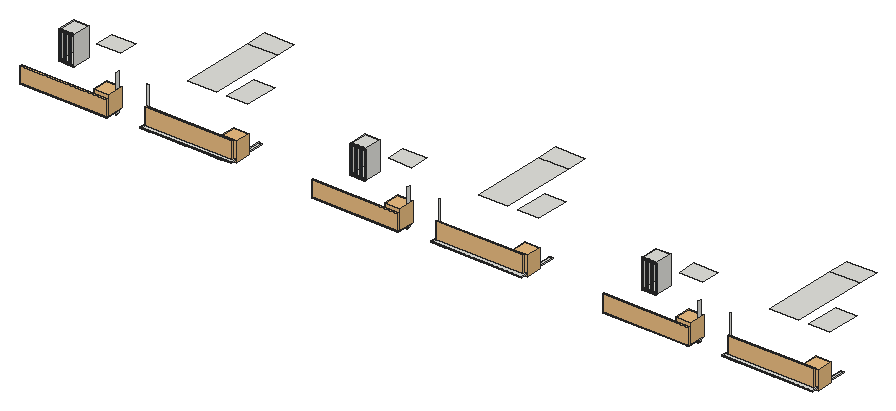
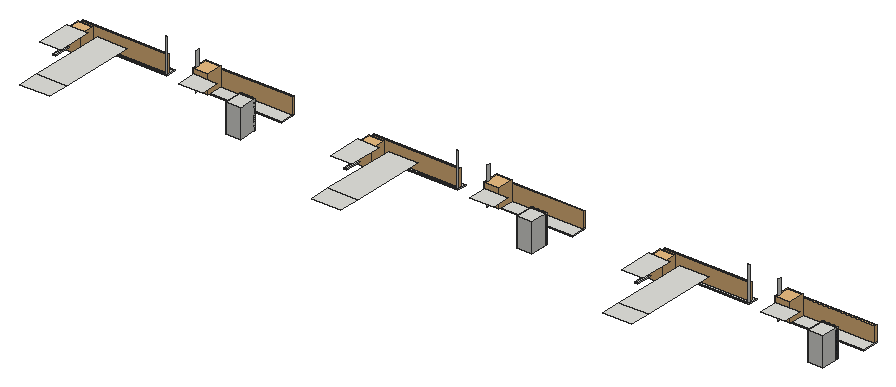
# SketchUp Ruby script. Lengths in inches.
U = 1.inch
M = Sketchup.active_model
def pt(a) = Geom::Point3d.new(a.map { |v| v * U })
def face(e, loops, mat)
  f = e.add_face(loops[0].map { |a| pt(a) })
  loops[1..].each { |l| e.add_face(l.map { |a| pt(a) }).erase! }
  f.material = f.back_material = mat if mat
  f
end
# faces: each face lists its corners as indices into pts; further lists are holes
def faces(e, pts, list, mat = nil) = list.each { |f| face(e, (f[0].is_a?(Array) ? f : [f]).map { |l| l.map { |i| pts[i] } }, mat) }
# xy, xz, yz: faces in a plane at the given z, y or x. An outline is a flat list of corners, or four numbers for a rectangle; further outlines are holes
def ring(l) = l.size == 4 ? [[l[0], l[1]], [l[2], l[1]], [l[2], l[3]], [l[0], l[3]]] : l.each_slice(2).to_a
def flat(e, list, mat, &to3) = list.each { |f| face(e, (f[0].is_a?(Array) ? f : [f]).map { |l| ring(l).map { |u, v| to3.(u, v) } }, mat) }
def xy(e, z, list, mat = nil) = flat(e, list, mat) { |x, y| [x, y, z] }
def xz(e, y, list, mat = nil) = flat(e, list, mat) { |x, z| [x, y, z] }
def yz(e, x, list, mat = nil) = flat(e, list, mat) { |y, z| [x, y, z] }
def lines(e, pts, list) = list.each { |a, b| e.add_line(pt(pts[a]), pt(pts[b])) }
# prism: a flat outline (further loops are holes) pulled along v
def prism(e, loops, v, mat = nil)
  f = face(e, loops, mat); d = Geom::Vector3d.new(v.map { |x| x * U })
  f.pushpull(f.normal.samedirection?(d) ? d.length : -d.length)
end
def box(e, o, s, mat = nil) = prism(e, [[o, [o[0] + s[0], o[1], o[2]], [o[0] + s[0], o[1] + s[1], o[2]], [o[0], o[1] + s[1], o[2]]]], [0, 0, s[2]], mat)
def at(x, y, z, deg = 0) = Geom::Transformation.translation(pt([x, y, z])) * Geom::Transformation.rotation(ORIGIN, Z_AXIS, deg.degrees)
def axes(o, x, y, z) = Geom::Transformation.new([*x, 0, *y, 0, *z, 0, *pt(o).to_a, 1])
def part(name) = M.definitions.add(name)
# library, detail: a bought-in or finely detailed component or shape, given as its bounding box
def library(name, o, s) = part(name).tap { |d| box(d.entities, o, s) }
def detail(e, o, s) = box(e.add_group.entities, o, s)
def put(e, d, t, mat = nil) = e.add_instance(d, t).tap { |i| i.material = mat if mat }
def group(e, t, mat = nil) = e.add_group.tap { |g| g.transformation = t; g.material = mat if mat }.entities
root = M.entities
M.materials.add("Wine2").color = [0, 0, 0]
M.materials["Wine2"].alpha = 0
M.materials.add("[0130_Gainsboro]").color = [39, 45, 50]
M.materials.add("[Wood Veneer 01]").color = [51, 28, 15]
c1 = library("plant (1)",[-35.72,-28.42,0],[66.31,67.39,84.38])
c2 = library("Glass Railing",[0,0,0],[139.5,4.76,42])
c3 = part("Group\#55")
xy(c3.entities,0,[[0,-0.98,43.07,0],[0,0,43.07,1.4]],"[0130_Gainsboro]")
xy(c3.entities,0.3,[[0.3,-1.43,42.77,-0.98]],"[0130_Gainsboro]")
xy(c3.entities,2.95,[[2.95,-1.43,40.12,-0.63],[2.95,-0.63,40.12,0],[2.95,0,40.12,0.64],[2.95,0.64,40.12,1.4]],"[0130_Gainsboro]")
xy(c3.entities,3.54,[[3.54,-0.63,39.53,0],[3.54,0,39.53,0.64]],"[0130_Gainsboro]")
xy(c3.entities,111.8125,[[3.54,-0.63,39.53,0],[3.54,0,39.53,0.64]],"[0130_Gainsboro]")
xy(c3.entities,112.4,[[2.95,-1.43,40.12,-0.63],[2.95,-0.63,40.12,0],[2.95,0,40.12,0.64],[2.95,0.64,40.12,1.4]],"[0130_Gainsboro]")
xy(c3.entities,115.05,[[0.3,-1.43,42.77,-0.98]],"[0130_Gainsboro]")
xy(c3.entities,115.35,[[0,-0.98,43.07,0],[0,0,43.07,1.4]],"[0130_Gainsboro]")
xz(c3.entities,-1.43,[[[0.3,0.3,42.77,115.05],[2.95,2.95,40.12,112.4]]],"[Wood Veneer 01]")
xz(c3.entities,-0.98,[[[0,0,43.07,115.35],[0.3,0.3,42.77,115.05]]],"[0130_Gainsboro]")
xz(c3.entities,-0.63,[[[2.95,2.95,40.12,112.4],[3.54,3.54,39.53,111.8125]]],"[0130_Gainsboro]")
xz(c3.entities,0,[[3.54,3.54,39.53,111.8125]],"Wine2")
xz(c3.entities,0,[[[0,0,43.07,115.35],[2.95,2.95,40.12,112.4]],[[2.95,2.95,40.12,112.4],[3.54,3.54,39.53,111.8125]]],"[0130_Gainsboro]")
xz(c3.entities,0.64,[[[2.95,2.95,40.12,112.4],[3.54,3.54,39.53,111.8125]]],"[0130_Gainsboro]")
xz(c3.entities,1.4,[[[0,0,43.07,115.35],[2.95,2.95,40.12,112.4]]],"[0130_Gainsboro]")
yz(c3.entities,0,[[-0.98,0,0,115.35],[0,0,1.4,115.35]],"[0130_Gainsboro]")
yz(c3.entities,0.3,[[-1.43,0.3,-0.98,115.05]],"[0130_Gainsboro]")
yz(c3.entities,2.95,[[-1.43,2.95,-0.63,112.4],[-0.63,2.95,0,112.4],[0,2.95,0.64,112.4],[0.64,2.95,1.4,112.4]],"[0130_Gainsboro]")
yz(c3.entities,3.54,[[-0.63,3.54,0,111.8125],[0,3.54,0.64,111.8125]],"[0130_Gainsboro]")
yz(c3.entities,39.53,[[-0.63,3.54,0,111.8125],[0,3.54,0.64,111.8125]],"[0130_Gainsboro]")
yz(c3.entities,40.12,[[-1.43,2.95,-0.63,112.4],[-0.63,2.95,0,112.4],[0,2.95,0.64,112.4],[0.64,2.95,1.4,112.4]],"[0130_Gainsboro]")
yz(c3.entities,42.77,[[-1.43,0.3,-0.98,115.05]],"[0130_Gainsboro]")
yz(c3.entities,43.07,[[-0.98,0,0,115.35],[0,0,1.4,115.35]],"[0130_Gainsboro]")
c4 = part("Component\#21")
put(c4.entities,c3,axes([90.57,1.43,0],[1.05148,0,0],[0,1,0],[0,0,1]))
put(c4.entities,c3,axes([0,1.43,0],[1.05148,0,0],[0,1,0],[0,0,1]))
put(c4.entities,c3,axes([45.29,1.43,0],[1.05148,0,0],[0,1,0],[0,0,1]),"[Wood Veneer 01]")
xy(root,409.375,[[315.43,286.21,315.68,293.45],[1049,286.21,1049.24,293.45],[1782.56,286.21,1782.8,293.45]])
xy(root,416.75,[[100.18,253.3,100.18,253.61,315.68,253.61,315.68,255.92,318.3,255.92,318.3,253.3],[833.74,253.3,833.74,253.61,1049.24,253.61,1049.24,255.92,1051.86,255.92,1051.86,253.3],[1567.3,253.3,1567.3,253.61,1782.8,253.61,1782.8,255.92,1785.43,255.92,1785.43,253.3],[100.18,253.61,315.68,293.45],[833.74,253.61,1049.24,293.45],
  [1567.3,253.61,1782.8,293.45],[315.68,255.92,318.3,293.45],[1049.24,255.92,1051.86,293.45],[1782.8,255.92,1785.43,293.45],[393.95,263.8,393.95,286.21,614.76,286.21,614.76,361.27,622,361.27,622,266.43,398.72,266.43,398.72,263.8],
  [398.72,263.8,404.72,266.43],[404.72,263.8,410.72,266.43],[410.72,263.8,416.72,266.43],[416.72,263.8,422.72,266.43],[422.72,263.8,428.72,266.43],
  [428.72,263.8,434.72,266.43],[434.72,263.8,440.72,266.43],[440.72,263.8,446.72,266.43],[446.72,263.8,452.72,266.43],[452.72,263.8,458.72,266.43],
  [458.72,263.8,464.72,266.43],[464.72,263.8,470.72,266.43],[470.72,263.8,476.72,266.43],[476.72,263.8,482.72,266.43],[482.72,263.8,488.72,266.43],
  [488.72,263.8,494.72,266.43],[494.72,263.8,500.72,266.43],[500.72,263.8,506.72,266.43],[506.72,263.8,512.72,266.43],[512.72,263.8,518.72,266.43],
  [518.72,263.8,524.72,266.43],[524.72,263.8,530.72,266.43],[530.72,263.8,536.72,266.43],[536.72,263.8,542.72,266.43],[542.72,263.8,548.72,266.43],
  [548.72,263.8,554.72,266.43],[554.72,263.8,560.72,266.43],[560.72,263.8,566.72,266.43],[566.72,263.8,572.72,266.43],[572.72,263.8,578.72,266.43],
  [578.72,263.8,584.72,266.43],[584.72,263.8,590.72,266.43],[590.72,263.8,596.72,266.43],[596.72,263.8,602.72,266.43],[602.72,263.8,608.72,266.43],
  [608.72,263.8,622,266.43],[1127.51,263.8,1127.51,286.21,1348.32,286.21,1348.32,361.27,1355.5625,361.27,1355.5625,266.43,1132.28,266.43,1132.28,263.8],[1132.28,263.8,1138.28,266.43],[1138.28,263.8,1144.28,266.43],[1144.28,263.8,1150.28,266.43],
  [1150.28,263.8,1156.28,266.43],[1156.28,263.8,1162.28,266.43],[1162.28,263.8,1168.28,266.43],[1168.28,263.8,1174.28,266.43],[1174.28,263.8,1180.28,266.43],
  [1180.28,263.8,1186.28,266.43],[1186.28,263.8,1192.28,266.43],[1192.28,263.8,1198.28,266.43],[1198.28,263.8,1204.28,266.43],[1204.28,263.8,1210.28,266.43],
  [1210.28,263.8,1216.28,266.43],[1216.28,263.8,1222.28,266.43],[1222.28,263.8,1228.28,266.43],[1228.28,263.8,1234.28,266.43],[1234.28,263.8,1240.28,266.43],
  [1240.28,263.8,1246.28,266.43],[1246.28,263.8,1252.28,266.43],[1252.28,263.8,1258.28,266.43],[1258.28,263.8,1264.28,266.43],[1264.28,263.8,1270.28,266.43],
  [1270.28,263.8,1276.28,266.43],[1276.28,263.8,1282.28,266.43],[1282.28,263.8,1288.28,266.43],[1288.28,263.8,1294.28,266.43],[1294.28,263.8,1300.28,266.43],
  [1300.28,263.8,1306.28,266.43],[1306.28,263.8,1312.28,266.43],[1312.28,263.8,1318.28,266.43],[1318.28,263.8,1324.28,266.43],[1324.28,263.8,1330.28,266.43],
  [1330.28,263.8,1336.28,266.43],[1336.28,263.8,1342.28,266.43],[1342.28,263.8,1355.5625,266.43],[1861.07,263.8,1861.07,286.21,2081.89,286.21,2081.89,361.27,2089.125,361.27,2089.125,266.43,1865.84,266.43,1865.84,263.8],[1865.84,263.8,1871.84,266.43],
  [1871.84,263.8,1877.84,266.43],[1877.84,263.8,1883.84,266.43],[1883.84,263.8,1889.84,266.43],[1889.84,263.8,1895.84,266.43],[1895.84,263.8,1901.84,266.43],
  [1901.84,263.8,1907.84,266.43],[1907.84,263.8,1913.84,266.43],[1913.84,263.8,1919.84,266.43],[1919.84,263.8,1925.84,266.43],[1925.84,263.8,1931.84,266.43],
  [1931.84,263.8,1937.84,266.43],[1937.84,263.8,1943.84,266.43],[1943.84,263.8,1949.84,266.43],[1949.84,263.8,1955.84,266.43],[1955.84,263.8,1961.84,266.43],
  [1961.84,263.8,1967.84,266.43],[1967.84,263.8,1973.84,266.43],[1973.84,263.8,1979.84,266.43],[1979.84,263.8,1985.84,266.43],[1985.84,263.8,1991.84,266.43],
  [1991.84,263.8,1997.84,266.43],[1997.84,263.8,2003.84,266.43],[2003.84,263.8,2009.84,266.43],[2009.84,263.8,2015.84,266.43],[2015.84,263.8,2021.84,266.43],
  [2021.84,263.8,2027.84,266.43],[2027.84,263.8,2033.84,266.43],[2033.84,263.8,2039.84,266.43],[2039.84,263.8,2045.84,266.43],[2045.84,263.8,2051.84,266.43],
  [2051.84,263.8,2057.84,266.43],[2057.84,263.8,2063.84,266.43],[2063.84,263.8,2069.84,266.43],[2069.84,263.8,2075.84,266.43],[2075.84,263.8,2089.125,266.43]])
xy(root,418.9375,[[100.18,253.3,318.3,293.45],[833.74,253.3,1051.86,293.45],[1567.3,253.3,1785.43,293.45],[393.95,263.8,622,263.8,622,361.27,614.76,361.27,614.76,286.21,393.95,286.21],[1127.51,263.8,1355.5625,263.8,1355.5625,361.27,1348.32,361.27,1348.32,286.21,1127.51,286.21],
  [1861.07,263.8,2089.125,263.8,2089.125,361.27,2081.89,361.27,2081.89,286.21,1861.07,286.21]])
xy(root,425.31,[[111.92,361.27,149.24,408.14],[845.49,361.27,882.8,408.14],[1579.05,361.27,1616.36,408.14]])
xy(root,495.625,[[435.49,361.27,509.74,551.2],[1169.05,361.27,1243.3,551.2],[1902.61,361.27,1976.86,551.2],[435.49,551.2,509.74,604.39],[1169.05,551.2,1243.3,604.39],
  [1902.61,551.2,1976.86,604.39]])
xy(root,495.6875,[[534.92,361.27,587.67,445.08],[1268.48,361.27,1321.23,445.08],[2002.05,361.27,2054.8,445.08]])
xy(root,497.42,[[207.81,361.27,266.47,408.14],[941.37,361.27,1000.03,408.14],[1674.93,361.27,1733.6,408.14]])
xy(root,497.43,[[111.92,361.27,149.24,408.14],[845.49,361.27,882.8,408.14],[1579.05,361.27,1616.36,408.14]])
xz(root,253.3,[[100.18,416.75,318.3,418.9375],[833.74,416.75,1051.86,418.9375],[1567.3,416.75,1785.43,418.9375]],"[Wood Veneer 01]")
xz(root,263.8,[[393.95,416.75,622,418.9375],[1127.51,416.75,1355.5625,418.9375],[1861.07,416.75,2089.125,418.9375]],"[Wood Veneer 01]")
xz(root,286.21,[[393.95,416.75,396.57,418.9375],[396.57,416.75,614.76,418.9375],[1127.51,416.75,1130.14,418.9375],[1130.14,416.75,1348.32,418.9375],[1861.07,416.75,1863.7,418.9375],
  [1863.7,416.75,2081.89,418.9375],[393.95,418.9375,396.57,505.3125],[1127.51,418.9375,1130.14,505.3125],[1861.07,418.9375,1863.7,505.3125]])
xz(root,293.45,[[315.43,409.375,315.68,416.75],[1049,409.375,1049.24,416.75],[1782.56,409.375,1782.8,416.75],[100.18,416.75,315.43,418.9375],[315.43,416.75,318.3,418.9375],
  [833.74,416.75,1049,418.9375],[1049,416.75,1051.86,418.9375],[1567.3,416.75,1782.56,418.9375],[1782.56,416.75,1785.43,418.9375]])
xz(root,361.27,[[614.76,416.75,622,418.9375],[1348.32,416.75,1355.5625,418.9375],[2081.89,416.75,2089.125,418.9375]])
xz(root,408.14,[[111.92,425.31,149.24,497.43],[845.49,425.31,882.8,497.43],[1579.05,425.31,1616.36,497.43]])
yz(root,100.18,[[253.3,416.75,293.45,418.9375]])
yz(root,111.92,[[361.27,425.31,408.14,497.43]])
yz(root,149.24,[[361.27,425.31,408.14,497.43]])
yz(root,315.43,[[286.21,409.375,293.45,503.875]])
yz(root,318.3,[[253.3,416.75,293.45,418.9375]])
yz(root,393.95,[[263.8,416.75,286.21,418.9375]])
yz(root,614.76,[[286.21,416.75,361.27,418.9375]])
yz(root,622,[[263.8,416.75,266.43,418.9375],[266.43,416.75,361.27,418.9375]])
yz(root,833.74,[[253.3,416.75,293.45,418.9375]])
yz(root,845.49,[[361.27,425.31,408.14,497.43]])
yz(root,882.8,[[361.27,425.31,408.14,497.43]])
yz(root,1049,[[286.21,409.375,293.45,503.875]])
yz(root,1051.86,[[253.3,416.75,293.45,418.9375]])
yz(root,1127.51,[[263.8,416.75,286.21,418.9375]])
yz(root,1348.32,[[286.21,416.75,361.27,418.9375]])
yz(root,1355.5625,[[263.8,416.75,266.43,418.9375],[266.43,416.75,361.27,418.9375]])
yz(root,1567.3,[[253.3,416.75,293.45,418.9375]])
yz(root,1579.05,[[361.27,425.31,408.14,497.43]])
yz(root,1616.36,[[361.27,425.31,408.14,497.43]])
yz(root,1782.56,[[286.21,409.375,293.45,503.875]])
yz(root,1785.43,[[253.3,416.75,293.45,418.9375]])
yz(root,1861.07,[[263.8,416.75,286.21,418.9375]])
yz(root,2081.89,[[286.21,416.75,361.27,418.9375]])
yz(root,2089.125,[[263.8,416.75,266.43,418.9375],[266.43,416.75,361.27,418.9375]])
put(root,c1,axes([1338.13,298.81,410.31],[0.57,0,0],[0,0.57,0],[0,0,0.57]))
put(root,c1,axes([2071.69,298.81,410.31],[0.57,0,0],[0,0.57,0],[0,0,0.57]))
put(root,c1,axes([604.57,298.81,410.31],[0.57,0,0],[0,0.57,0],[0,0,0.57]))
put(root,c2,axes([833.74,253.3,416.75],[1.55814,0,0],[0,1,0],[0,0,1]))
put(root,c2,axes([1567.3,253.3,416.75],[1.55814,0,0],[0,1,0],[0,0,1]))
put(root,c2,axes([100.18,253.3,416.75],[1.55814,0,0],[0,1,0],[0,0,1]))
put(root,c2,axes([1131.22,275.08,417.62],[1.55814,0,0],[0,1,0],[0,0,1]))
put(root,c2,axes([1864.78,275.08,417.62],[1.55814,0,0],[0,1,0],[0,0,1]))
put(root,c2,axes([397.65,275.08,417.62],[1.55814,0,0],[0,1,0],[0,0,1]))
put(root,c1,axes([1034.43,276.71,418.9375],[0.57,0,0],[0,0.57,0],[0,0,0.57]))
put(root,c1,axes([1767.99,276.71,418.9375],[0.57,0,0],[0,0.57,0],[0,0,0.57]))
put(root,c1,axes([300.87,276.71,418.9375],[0.57,0,0],[0,0.57,0],[0,0,0.57]))
put(root,c4,axes([845.49,361.27,425.31],[0.27464,0,0],[0,1.2771,0],[0,0,0.62578]))
put(root,c4,axes([1579.05,361.27,425.31],[0.27464,0,0],[0,1.2771,0],[0,0,0.62578]))
put(root,c4,axes([111.92,361.27,425.31],[0.27464,0,0],[0,1.2771,0],[0,0,0.62578]))
